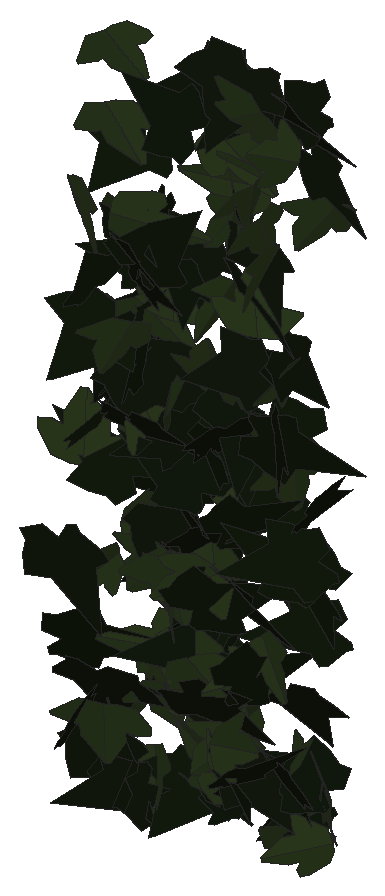
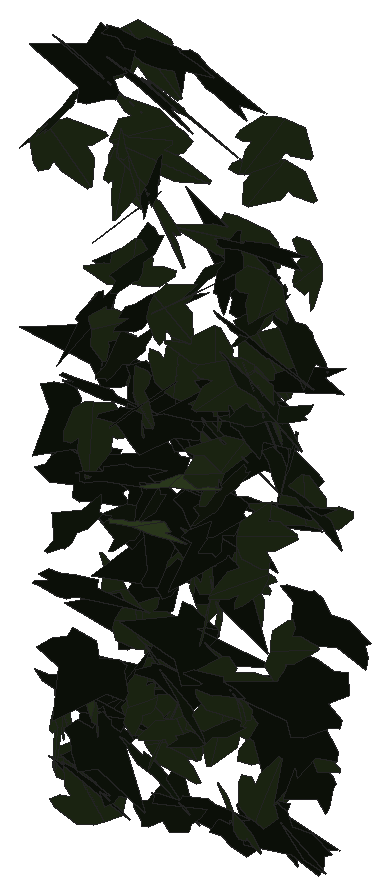
# SketchUp Ruby script. Lengths in inches.
U = 1.inch
M = Sketchup.active_model
def pt(a) = Geom::Point3d.new(a.map { |v| v * U })
def face(e, loops, mat)
  f = e.add_face(loops[0].map { |a| pt(a) })
  loops[1..].each { |l| e.add_face(l.map { |a| pt(a) }).erase! }
  f.material = f.back_material = mat if mat
  f
end
# faces: each face lists its corners as indices into pts; further lists are holes
def faces(e, pts, list, mat = nil) = list.each { |f| face(e, (f[0].is_a?(Array) ? f : [f]).map { |l| l.map { |i| pts[i] } }, mat) }
# xy, xz, yz: faces in a plane at the given z, y or x. An outline is a flat list of corners, or four numbers for a rectangle; further outlines are holes
def ring(l) = l.size == 4 ? [[l[0], l[1]], [l[2], l[1]], [l[2], l[3]], [l[0], l[3]]] : l.each_slice(2).to_a
def flat(e, list, mat, &to3) = list.each { |f| face(e, (f[0].is_a?(Array) ? f : [f]).map { |l| ring(l).map { |u, v| to3.(u, v) } }, mat) }
def xy(e, z, list, mat = nil) = flat(e, list, mat) { |x, y| [x, y, z] }
def xz(e, y, list, mat = nil) = flat(e, list, mat) { |x, z| [x, y, z] }
def yz(e, x, list, mat = nil) = flat(e, list, mat) { |y, z| [x, y, z] }
def lines(e, pts, list) = list.each { |a, b| e.add_line(pt(pts[a]), pt(pts[b])) }
# prism: a flat outline (further loops are holes) pulled along v
def prism(e, loops, v, mat = nil)
  f = face(e, loops, mat); d = Geom::Vector3d.new(v.map { |x| x * U })
  f.pushpull(f.normal.samedirection?(d) ? d.length : -d.length)
end
def box(e, o, s, mat = nil) = prism(e, [[o, [o[0] + s[0], o[1], o[2]], [o[0] + s[0], o[1] + s[1], o[2]], [o[0], o[1] + s[1], o[2]]]], [0, 0, s[2]], mat)
def at(x, y, z, deg = 0) = Geom::Transformation.translation(pt([x, y, z])) * Geom::Transformation.rotation(ORIGIN, Z_AXIS, deg.degrees)
def axes(o, x, y, z) = Geom::Transformation.new([*x, 0, *y, 0, *z, 0, *pt(o).to_a, 1])
def part(name) = M.definitions.add(name)
# library, detail: a bought-in or finely detailed component or shape, given as its bounding box
def library(name, o, s) = part(name).tap { |d| box(d.entities, o, s) }
def detail(e, o, s) = box(e.add_group.entities, o, s)
def put(e, d, t, mat = nil) = e.add_instance(d, t).tap { |i| i.material = mat if mat }
def group(e, t, mat = nil) = e.add_group.tap { |g| g.transformation = t; g.material = mat if mat }.entities
root = M.entities
M.materials.add("1026 AP 7946 SUNNY SIDE UP").color = [254, 231, 186]
M.materials.add("efeu1").color = [18, 25, 13]
M.materials.add("efeu2").color = [43, 57, 29]
c1 = part("ivyleaf_9")
p = [[1.54,2.16,1.25],[1.36,2.04,1.19],[-0.21,0.99,0.68],[-0.71,1.11,0.82],[-0.85,0.86,0.67],[-0.8,0.17,0.21],
  [-0.9,-0.01,0.1],[-0.67,-0.16,-0.02],[-0.08,-0.08,-0.05],[-0.03,-0.6,-0.4],[0.65,-0.88,-0.66],[0.83,-0.6,-0.49],
  [1.29,-0.42,-0.43],[1.8125,-0.07,-0.26],[1.21,0.44,0.15]]
faces(c1.entities,p,[[0,1,2,3,4,5,6,7,8,9,10,11,12,13,14]],"efeu1")
c2 = part("ivyleaf_10")
p = [[0,0.5,-0.03],[-0.0625,2.02,-0.43],[-0.19,2.01,-0.46],[-0.54,1.05,-0.29],[-0.52,0.625,-0.18],[-0.83,0.76,-0.28],
  [-1.16,0.64,-0.33],[-1.15,0.33,-0.24],[-0.77,-0.39,0.02],[-0.3,-0.51,0.16],[0.04,-0.48,0.23],[-0.02,2.01,-0.4375],
  [-0.06,2.01,-0.43],[0.04,-0.49,0.23],[0.67,-0.49,0.14],[1.38,0.36,-0.2],[1.375,0.51,-0.24],[0.81,0.65,-0.19],
  [0.62,0.59,-0.15],[0.6,1.09,-0.28],[0.5,1.23,-0.31]]
faces(c2.entities,p,[[0,1,2,3,4,5,6,7,8,9,10],[11,12,0,13,14,15,16,17,18,19,20]],"efeu2")
put(root,c1,axes([144.02,211.13,286.05],[0.051,-0.0466,-0.38106],[0.48121,-0.20826,0.05349],[-0.33408,-0.30709,0.01888]),"1026 AP 7946 SUNNY SIDE UP")
put(root,c1,axes([142.66,210.79,290.45],[-0.41002,0.00525,-0.29295],[-0.44658,0.01655,0.26868],[0.02475,0.38549,-0.00529]),"1026 AP 7946 SUNNY SIDE UP")
put(root,c2,axes([143.42,210.64,280.99],[-0.03526,0.16378,0.34753],[-0.07787,0.33276,-0.16835],[-0.58316,-0.05434,0.00147]),"1026 AP 7946 SUNNY SIDE UP")
put(root,c2,axes([143.85,211.09,288.69],[0.13652,-0.34131,0.17691],[0.06301,-0.169,-0.3638],[0.59885,0.09559,-0.00205]),"1026 AP 7946 SUNNY SIDE UP")
put(root,c1,axes([143.42,210.74,280.36],[0.16891,0.33769,-0.08584],[0.01032,0.08722,0.36501],[0.54754,-0.10582,0.0196]),"1026 AP 7946 SUNNY SIDE UP")
put(root,c2,axes([141.375,211.02,286.71],[-0.25952,-0.30703,0.11261],[-0.06423,-0.10404,-0.35948],[0.50935,-0.16955,0.01205]),"1026 AP 7946 SUNNY SIDE UP")
put(root,c2,axes([144.08,211.18,290.28],[-0.01561,0.17803,0.34127],[0.06022,-0.32817,0.18151],[0.58687,0.03841,-0.00955]),"1026 AP 7946 SUNNY SIDE UP")
put(root,c2,axes([141.08,210.96,280.56],[-0.55199,-0.18292,0.00641],[0.01698,-0.03637,-0.4062],[0.28735,-0.34923,0.03632]),"1026 AP 7946 SUNNY SIDE UP")
put(root,c1,axes([143.14,211.19,280.37],[0.06729,-0.26436,0.21998],[0.07612,-0.20981,-0.27687],[0.53039,0.06365,0.01183]),"1026 AP 7946 SUNNY SIDE UP")
put(root,c1,axes([140.21,211.05,282.93],[-0.25952,-0.09043,-0.37086],[0.54319,0.10514,-0.19003],[0.21132,-0.38132,0.03302]),"1026 AP 7946 SUNNY SIDE UP")
put(root,c1,axes([141.36,211.19,287.61],[0.18886,-0.16012,0.31476],[0.21959,-0.2743,-0.20565],[0.49735,0.18192,-0.02872]),"1026 AP 7946 SUNNY SIDE UP")
put(root,c2,axes([142.77,211.04,283.27],[0.43211,-0.0276,-0.24252],[-0.37047,0.00526,-0.28414],[0.03836,0.36171,-0.01225]),"1026 AP 7946 SUNNY SIDE UP")
put(root,c1,axes([142.77,210.87,282.84],[0.00919,0.02174,0.39223],[0.59548,0.04342,-0.00829],[-0.06889,0.37817,-0.01935]),"1026 AP 7946 SUNNY SIDE UP")
put(root,c2,axes([141.98,211.29,282.53],[0.00162,-0.02873,-0.38292],[0.14518,-0.35993,0.02683],[-0.56767,-0.09213,0.00577]),"1026 AP 7946 SUNNY SIDE UP")
put(root,c1,axes([142.73,210.95,284.68],[-0.10724,0.15198,0.33389],[-0.479,0.14708,-0.1366],[-0.29327,-0.29581,0.10101]),"1026 AP 7946 SUNNY SIDE UP")
put(root,c1,axes([140.63,210.72,280.29],[0.06819,0.18704,0.34131],[0.17457,0.3116,-0.19501],[-0.57067,0.11767,-0.01887]),"1026 AP 7946 SUNNY SIDE UP")
put(root,c1,axes([140.89,211.33,286.51],[-0.40385,-0.2696,0.15117],[-0.13022,-0.12544,-0.38349],[0.46594,-0.26873,0.02385]),"1026 AP 7946 SUNNY SIDE UP")
put(root,c1,axes([144.55,211.23,284.06],[-0.48677,-0.03035,0.18876],[-0.27841,-0.06036,-0.31854],[0.08903,-0.35472,0.03591]),"1026 AP 7946 SUNNY SIDE UP")
put(root,c2,axes([143.46,211.32,281.8125],[-0.12307,-0.01797,0.34416],[-0.11811,-0.3335,-0.03855],[0.5128,-0.08112,0.07372]),"1026 AP 7946 SUNNY SIDE UP")
put(root,c1,axes([141.66,211.03,287.88],[-0.264,0.21162,0.30055],[0.33459,-0.19993,0.27552],[0.4555,0.2695,-0.02819]),"1026 AP 7946 SUNNY SIDE UP")
put(root,c1,axes([143.41,211.36,286.61],[-0.23239,-0.10983,0.32218],[-0.32126,-0.2403,-0.18744],[0.41158,-0.24958,0.0356]),"1026 AP 7946 SUNNY SIDE UP")
put(root,c1,axes([142.57,210.93,281.4],[0.55612,0.11164,0.10887],[0.17566,-0.00682,-0.38004],[-0.16506,0.36889,-0.03762]),"1026 AP 7946 SUNNY SIDE UP")
put(root,c1,axes([141.49,211.3,279.44],[-0.04792,-0.05968,-0.36006],[-0.17902,-0.33021,0.06645],[-0.52743,0.1175,0.01016]),"1026 AP 7946 SUNNY SIDE UP")
put(root,c2,axes([142.125,211.13,283.13],[-0.58142,-0.15639,-0.04207],[0.10036,-0.04996,-0.40746],[0.23312,-0.36855,0.0705]),"1026 AP 7946 SUNNY SIDE UP")
put(root,c1,axes([143.48,211.08,280.49],[0.07023,-0.24147,-0.25612],[-0.02756,0.24739,-0.25073],[0.54272,0.04381,0.02041]),"1026 AP 7946 SUNNY SIDE UP")
put(root,c1,axes([142.32,211.14,285.36],[-0.46374,0.23477,0.0162],[-0.04516,-0.01304,-0.38734],[-0.36708,-0.29499,0.02719]),"1026 AP 7946 SUNNY SIDE UP")
put(root,c1,axes([140.38,210.98,281.5],[0.28045,0.07021,0.36112],[0.54911,0.04756,-0.1928],[-0.11743,0.39006,-0.03911]),"1026 AP 7946 SUNNY SIDE UP")
put(root,c1,axes([143.77,211.09,285.82],[0.25466,-0.00531,-0.33978],[0.39086,0.24346,0.12314],[0.3409,-0.27518,0.11263]),"1026 AP 7946 SUNNY SIDE UP")
put(root,c2,axes([140.34,211.27,288.4375],[-0.29347,0.24032,-0.2328],[0.17324,-0.20097,-0.31322],[-0.49048,-0.21478,0.02867]),"1026 AP 7946 SUNNY SIDE UP")
put(root,c1,axes([143.08,211.11,285.68],[-0.02537,0.337,-0.14455],[0.02424,-0.14162,-0.3483],[-0.57465,-0.02085,-0.00831]),"1026 AP 7946 SUNNY SIDE UP")
put(root,c1,axes([141.52,211.01,285.35],[0.61771,0.06958,-0.10511],[-0.16737,0.0157,-0.40951],[-0.09946,0.40567,0.03632]),"1026 AP 7946 SUNNY SIDE UP")
put(root,c1,axes([140.87,211.11,285.11],[-0.26971,0.33859,-0.04449],[0.00492,-0.04892,-0.3908],[-0.53708,-0.17048,0.01877]),"1026 AP 7946 SUNNY SIDE UP")
put(root,c1,axes([140.87,211.07,281.08],[0.50651,0.17273,-0.1679],[-0.21959,-0.08641,-0.37693],[-0.30334,0.35097,-0.0075]),"1026 AP 7946 SUNNY SIDE UP")
put(root,c2,axes([141.87,211.23,283.17],[-0.50382,-0.04345,0.19818],[-0.28559,-0.07919,-0.33012],[0.12181,-0.36537,0.04571]),"1026 AP 7946 SUNNY SIDE UP")
put(root,c2,axes([143.58,211.33,282.29],[0.32351,-0.07386,0.27122],[0.38296,-0.10143,-0.22562],[0.19684,0.31871,-0.0068]),"1026 AP 7946 SUNNY SIDE UP")
put(root,c2,axes([142.6875,211.27,283.47],[0.53836,-0.02327,0.11009],[0.16537,-0.02786,-0.35311],[0.04791,0.35762,-0.01824]),"1026 AP 7946 SUNNY SIDE UP")
put(root,c2,axes([143.51,211.18,290.8],[-0.37943,0.02082,0.30069],[-0.45991,-0.02122,-0.24777],[0.00492,-0.37802,0.02824]),"1026 AP 7946 SUNNY SIDE UP")
put(root,c2,axes([143.08,211.34,280.67],[-0.35285,-0.16502,0.22702],[-0.20863,-0.18562,-0.28228],[0.38065,-0.25471,0.05572]),"1026 AP 7946 SUNNY SIDE UP")
put(root,c2,axes([144.41,211.46,279.41],[-0.10226,0.00253,0.34629],[-0.12064,-0.33343,-0.01466],[0.51459,-0.07767,0.06538]),"1026 AP 7946 SUNNY SIDE UP")
put(root,c2,axes([142.55,211.19,281.69],[-0.45704,-0.11165,-0.21684],[0.33498,0.02467,-0.31737],[0.16578,-0.35765,0.04349]),"1026 AP 7946 SUNNY SIDE UP")
put(root,c1,axes([141.97,211.5,287.78],[-0.00831,-0.32593,0.16601],[0.01055,-0.16307,-0.33666],[0.5729,-0.00172,0.0086]),"1026 AP 7946 SUNNY SIDE UP")
put(root,c1,axes([144.41,211.3125,283.64],[-0.0171,0.06942,0.37548],[-0.58225,0.01365,-0.01399],[-0.02509,-0.36398,0.06888]),"1026 AP 7946 SUNNY SIDE UP")
put(root,c2,axes([142.18,211.01,285.72],[0.15723,-0.04257,0.3662],[-0.32599,0.2943,0.09805],[-0.4594,-0.22341,0.05575]),"1026 AP 7946 SUNNY SIDE UP")
put(root,c1,axes([142.76,211.16,285.22],[0.05396,-0.00324,-0.36796],[-0.56156,-0.00564,-0.03533],[-0.00834,0.35876,-0.00178]),"1026 AP 7946 SUNNY SIDE UP")
put(root,c1,axes([143.35,211,281.8],[0.05904,0.07713,0.3889],[0.50163,0.2057,-0.07487],[-0.33855,0.31824,-0.04312]),"1026 AP 7946 SUNNY SIDE UP")
put(root,c1,axes([142.52,211.46,281.875],[-0.0717,-0.11857,-0.3305],[-0.20961,-0.29116,0.12895],[-0.49419,0.1407,-0.00674]),"1026 AP 7946 SUNNY SIDE UP")
put(root,c1,axes([141.24,211.27,284.28],[-0.4652,-0.17399,-0.0994],[-0.15413,-0.02097,0.35207],[-0.27137,0.31018,-0.02956]),"1026 AP 7946 SUNNY SIDE UP")
put(root,c1,axes([142.75,211.1875,283.95],[0.06618,0.33439,-0.1291],[-0.01721,-0.12683,-0.34791],[-0.56229,0.04324,-0.00455]),"1026 AP 7946 SUNNY SIDE UP")
put(root,c2,axes([142.97,211.24,279.98],[-0.07722,0.39391,-0.00226],[0.00645,0.00498,0.40894],[0.61939,0.04905,-0.00454]),"1026 AP 7946 SUNNY SIDE UP")
put(root,c2,axes([141.33,211.23,288.39],[-0.04543,-0.0261,-0.40547],[0.61934,0.01633,-0.03082],[0.02867,-0.39416,0.02325]),"1026 AP 7946 SUNNY SIDE UP")
put(root,c1,axes([143.89,211.24,280.55],[0.4845,-0.10162,-0.14324],[-0.22619,0.00272,-0.3318],[0.14758,0.3378,-0.03827]),"1026 AP 7946 SUNNY SIDE UP")
put(root,c2,axes([140.5,211.2,284.4375],[0.53923,0.21013,-0.0385],[0.0204,0.05231,0.41282],[0.33531,-0.34111,0.0368]),"1026 AP 7946 SUNNY SIDE UP")
put(root,c1,axes([143.08,211.1,284.08],[0.0469,0.02991,0.35185],[0.47544,0.15895,-0.04063],[-0.25357,0.30357,-0.01111]),"1026 AP 7946 SUNNY SIDE UP")
put(root,c1,axes([140.85,211.01,287.25],[-0.00642,0.31856,0.26985],[-0.06591,0.25846,-0.32525],[-0.64333,-0.02966,0.03063]),"1026 AP 7946 SUNNY SIDE UP")
put(root,c2,axes([143.01,211.23,280.07],[-0.34385,0.07316,-0.33261],[-0.44514,0.16021,0.23556],[0.27107,0.35589,-0.03508]),"1026 AP 7946 SUNNY SIDE UP")
put(root,c2,axes([142.11,211.38,281.88],[0.44987,0.02204,0.22094],[0.33877,-0.03491,-0.29276],[0.00537,0.35578,-0.04031]),"1026 AP 7946 SUNNY SIDE UP")
put(root,c1,axes([141.99,211.27,283.11],[0.16238,0.05066,-0.35441],[-0.51662,-0.10422,-0.11793],[-0.18043,0.34402,0.0187]),"1026 AP 7946 SUNNY SIDE UP")
put(root,c1,axes([141.19,211.2,279.49],[-0.27982,0.01122,-0.32514],[-0.49487,0.02466,0.18382],[0.04244,0.36154,-0.00032]),"1026 AP 7946 SUNNY SIDE UP")
put(root,c1,axes([142.75,211.32,283.08],[0.52171,-0.11935,0.08438],[0.10698,-0.05414,-0.36249],[0.20159,0.3376,-0.02602]),"1026 AP 7946 SUNNY SIDE UP")
put(root,c2,axes([143.35,211.3,289.46],[-0.10227,-0.36453,-0.09857],[0.01663,0.09319,-0.38087],[0.59155,-0.06564,-0.00633]),"1026 AP 7946 SUNNY SIDE UP")
put(root,c2,axes([141.47,211.5625,281.43],[-0.16097,-0.03073,-0.33666],[0.2448,-0.30572,-0.02243],[-0.45406,-0.15393,0.10726]),"1026 AP 7946 SUNNY SIDE UP")
put(root,c1,axes([141.39,211.1,285.83],[0.05535,0.05877,0.38859],[-0.03951,0.378,-0.05609],[-0.59844,-0.01952,0.03964]),"1026 AP 7946 SUNNY SIDE UP")
put(root,c2,axes([140.875,211.39,289.8],[-0.46187,-0.14137,-0.13593],[0.25038,-0.04303,-0.31987],[0.17102,-0.31879,0.10119]),"1026 AP 7946 SUNNY SIDE UP")
put(root,c1,axes([141.66,211.62,283.98],[0.13639,-0.18769,0.30475],[0.18906,-0.27147,-0.21458],[0.51893,0.14823,-0.00193]),"1026 AP 7946 SUNNY SIDE UP")
put(root,c1,axes([143.05,211.59,291.125],[-0.57566,-0.14397,-0.13555],[0.21247,0.01216,-0.40348],[0.21995,-0.38856,0.035]),"1026 AP 7946 SUNNY SIDE UP")
put(root,c2,axes([140.65,211.64,282.52],[0.01769,0.11224,-0.32719],[-0.19676,-0.29433,-0.11322],[-0.49279,0.12155,0.03346]),"1026 AP 7946 SUNNY SIDE UP")
put(root,c1,axes([142.875,211.7,285.63],[-0.06354,-0.3982,0.12132],[-0.0195,-0.11938,-0.41302],[0.65366,-0.04227,-0.00053]),"1026 AP 7946 SUNNY SIDE UP")
put(root,c2,axes([143.5,211.34,288.99],[-0.11298,-0.33498,-0.17481],[0.08331,0.16004,-0.35161],[0.58319,-0.08776,0.01636]),"1026 AP 7946 SUNNY SIDE UP")
put(root,c2,axes([141.74,211.63,281.52],[0.04735,0.07295,0.39459],[-0.34418,-0.31425,0.07763],[0.50659,-0.22032,0.01586]),"1026 AP 7946 SUNNY SIDE UP")
put(root,c1,axes([140.54,211.5,279.72],[-0.15834,-0.11435,-0.36878],[0.52328,0.14358,-0.14311],[0.27235,-0.34235,0.06058]),"1026 AP 7946 SUNNY SIDE UP")
put(root,c1,axes([143.2,211.32,279.78],[-0.22871,0.27485,0.14026],[-0.16319,0.09589,-0.31672],[-0.4527,-0.17343,0.04331]),"1026 AP 7946 SUNNY SIDE UP")
put(root,c2,axes([141.6,211.35,285.19],[0.24986,0.33106,0.13706],[0.09988,0.11497,-0.37756],[-0.55094,0.17099,-0.00629]),"1026 AP 7946 SUNNY SIDE UP")
put(root,c1,axes([142.79,211.31,282.89],[-0.09054,-0.15315,0.32786],[0.33347,0.24394,0.16145],[-0.44563,0.21366,0.0542]),"1026 AP 7946 SUNNY SIDE UP")
put(root,c2,axes([143.08,211.73,280.88],[0.00484,0.07556,-0.37536],[-0.14634,-0.35308,-0.07822],[-0.5672,0.09174,0.01698]),"1026 AP 7946 SUNNY SIDE UP")
put(root,c1,axes([141.33,211.33,286.04],[0.16389,-0.16952,-0.39179],[0.24798,0.37797,-0.12715],[0.60444,-0.1091,0.1584]),"1026 AP 7946 SUNNY SIDE UP")
put(root,c2,axes([143.73,211.72,286.52],[-0.11059,0.09845,-0.34105],[-0.14968,-0.33085,-0.08232],[-0.52293,0.07388,0.09569]),"1026 AP 7946 SUNNY SIDE UP")
put(root,c2,axes([141.75,211.45,281],[-0.34505,-0.2505,-0.08079],[0.10243,0.04514,-0.34227],[0.39914,-0.22814,0.01799]),"1026 AP 7946 SUNNY SIDE UP")
put(root,c1,axes([144.5,211.43,280.375],[-0.27519,0.15239,0.29296],[-0.41616,0.11552,-0.2316],[-0.28802,-0.31251,0.05473]),"1026 AP 7946 SUNNY SIDE UP")
put(root,c1,axes([141.74,211.34,283.86],[0.04925,-0.19291,-0.34576],[-0.08218,0.33043,-0.1994],[0.60163,0.06093,0.00106]),"1026 AP 7946 SUNNY SIDE UP")
put(root,c2,axes([141.35,211.64,279.65],[0.3925,-0.13871,0.22623],[0.26912,-0.14269,-0.29306],[0.30859,0.30086,-0.03217]),"1026 AP 7946 SUNNY SIDE UP")
put(root,c1,axes([142.78,211.77,288.89],[-0.01028,-0.04722,0.38112],[-0.02286,-0.36996,-0.05105],[0.58641,-0.01525,0.00469]),"1026 AP 7946 SUNNY SIDE UP")
put(root,c1,axes([142.23,211.7,279.61],[-0.51481,-0.1495,-0.01446],[0.03993,-0.02399,-0.36943],[0.23259,-0.32679,0.03141]),"1026 AP 7946 SUNNY SIDE UP")
put(root,c1,axes([141.25,211.7,286.125],[-0.35429,0.10957,-0.26929],[0.24121,-0.23452,-0.2383],[-0.37582,-0.25381,0.10091]),"1026 AP 7946 SUNNY SIDE UP")
put(root,c1,axes([143.18,211.7,288.43],[0.08584,-0.36796,0.01992],[-0.0033,-0.02197,-0.38331],[0.57955,0.05437,-0.00513]),"1026 AP 7946 SUNNY SIDE UP")
put(root,c1,axes([143,211.6875,287.76],[0.26216,-0.30471,0.11327],[0.07591,-0.10087,-0.35837],[0.50462,0.17348,-0.00494]),"1026 AP 7946 SUNNY SIDE UP")
put(root,c2,axes([143.33,211.46,287.32],[0.44377,0.22803,-0.01343],[-0.01209,0.03224,0.37271],[0.35906,-0.28074,0.02915]),"1026 AP 7946 SUNNY SIDE UP")
put(root,c2,axes([143.15,211.55,289.39],[0.11412,-0.01954,-0.37672],[-0.57044,0.04612,-0.07647],[0.07716,0.36984,-0.00816]),"1026 AP 7946 SUNNY SIDE UP")
put(root,c2,axes([142.46,211.57,286],[-0.55879,0.07283,0.00569],[0.01663,0.02623,0.37276],[0.11359,0.35444,-0.02658]),"1026 AP 7946 SUNNY SIDE UP")
put(root,c1,axes([142.51,211.79,279.3],[-0.29881,-0.11665,0.21323],[0.15892,-0.28003,-0.06841],[0.33909,0.02846,0.21996]),"1026 AP 7946 SUNNY SIDE UP")
put(root,c2,axes([140.96,211.61,286.47],[0.2475,-0.32145,-0.03347],[-0.05134,0.0181,-0.36796],[0.50514,0.15934,-0.021]),"1026 AP 7946 SUNNY SIDE UP")
put(root,c1,axes([140.32,211.86,285.48],[0.14373,-0.16966,-0.31945],[0.40744,-0.18428,0.18205],[-0.37607,-0.2645,0.07515]),"1026 AP 7946 SUNNY SIDE UP")
put(root,c2,axes([142.72,211.55,289.91],[0.36052,0.10019,0.28471],[0.41221,0.08731,-0.25668],[-0.20729,0.34787,-0.01524]),"1026 AP 7946 SUNNY SIDE UP")
put(root,c1,axes([142.94,211.77,283.79],[0.23117,-0.32702,0.12823],[0.0777,-0.11629,-0.37004],[0.54573,0.15508,-0.00163]),"1026 AP 7946 SUNNY SIDE UP")
put(root,c1,axes([141.4,211.83,288.35],[-0.08349,0.02961,-0.38672],[0.41402,-0.26833,-0.06171],[-0.42364,-0.26807,0.0159]),"1026 AP 7946 SUNNY SIDE UP")
put(root,c1,axes([141.92,211.59,284.37],[0.03254,0.03646,-0.36137],[-0.49739,-0.1539,-0.03658],[-0.2459,0.31612,0.02618]),"1026 AP 7946 SUNNY SIDE UP")
put(root,c1,axes([144.02,211.8125,283.26],[0.07951,-0.29338,0.17226],[0.0944,-0.16027,-0.3063],[0.52385,0.07341,0.02905]),"1026 AP 7946 SUNNY SIDE UP")
put(root,c2,axes([141.98,211.4375,282.45],[-0.05873,0.31928,-0.18854],[-0.02374,0.1843,0.33219],[0.57961,0.0399,-0.0055]),"1026 AP 7946 SUNNY SIDE UP")
put(root,c1,axes([142.8125,211.74,285.41],[-0.31,-0.25942,-0.17623],[0.20745,0.11163,-0.33327],[0.44099,-0.23488,0.03289]),"1026 AP 7946 SUNNY SIDE UP")
put(root,c2,axes([140.83,211.85,280.08],[-0.09547,-0.23564,-0.27663],[-0.11206,-0.25753,0.24916],[-0.54885,0.09357,-0.00275]),"1026 AP 7946 SUNNY SIDE UP")
put(root,c2,axes([144.59,211.45,280.13],[-0.24183,0.26655,0.23286],[-0.23833,0.16983,-0.31368],[-0.49346,-0.21265,0.03738]),"1026 AP 7946 SUNNY SIDE UP")
put(root,c1,axes([144.39,211.33,284.72],[0.11147,0.23196,0.28815],[0.18773,0.25287,-0.2469],[-0.53796,0.13631,-0.02645]),"1026 AP 7946 SUNNY SIDE UP")
put(root,c1,axes([141.69,211.81,280.875],[0.05488,-0.31337,0.07481],[0.22733,-0.05163,-0.2942],[0.45255,0.06394,0.13871]),"1026 AP 7946 SUNNY SIDE UP")
put(root,c2,axes([142.46,211.85,287.33],[-0.05614,-0.30345,0.21902],[0.04387,-0.2169,-0.31284],[0.58251,-0.01291,0.04467]),"1026 AP 7946 SUNNY SIDE UP")
put(root,c1,axes([143.1,211.77,290.67],[-0.55155,0.05026,-0.09198],[0.12999,-0.05099,-0.36329],[-0.09583,-0.35841,0.0366]),"1026 AP 7946 SUNNY SIDE UP")
put(root,c2,axes([142.28,211.73,280.81],[0.36454,0.23218,-0.11321],[-0.10396,-0.09094,-0.33811],[-0.39121,0.24051,-0.01564]),"1026 AP 7946 SUNNY SIDE UP")
put(root,c1,axes([140.73,211.84,287.74],[0.15453,-0.33589,0.09597],[0.0357,-0.0924,-0.36105],[0.54774,0.10079,-0.00354]),"1026 AP 7946 SUNNY SIDE UP")
put(root,c2,axes([140.88,211.65,288.09],[-0.4996,0.16549,-0.01485],[-0.00108,-0.03444,-0.36789],[-0.26133,-0.31623,0.02991]),"1026 AP 7946 SUNNY SIDE UP")
put(root,c2,axes([142.72,211.67,288.7],[0.3398,-0.27306,-0.13555],[-0.15326,0.0884,-0.35762],[0.45017,0.2362,-0.01944]),"1026 AP 7946 SUNNY SIDE UP")
put(root,c1,axes([143.45,211.79,290.57],[0.32066,-0.17626,0.25433],[0.29999,-0.15829,-0.27858],[0.37246,0.27923,0.00543]),"1026 AP 7946 SUNNY SIDE UP")
put(root,c1,axes([143.41,211.92,284.44],[-0.39748,-0.20662,0.0875],[-0.0629,-0.08609,-0.33431],[0.34631,-0.25279,0.03971]),"1026 AP 7946 SUNNY SIDE UP")
put(root,c2,axes([144.5625,211.45,280.32],[0.06945,-0.00994,-0.38505],[-0.20752,0.35166,-0.02365],[0.54998,0.13394,0.0397]),"1026 AP 7946 SUNNY SIDE UP")
put(root,c2,axes([144.34,211.83,289.28],[-0.27462,-0.27186,0.16814],[-0.12118,-0.14617,-0.33348],[0.48494,-0.19048,0.01189]),"1026 AP 7946 SUNNY SIDE UP")
put(root,c2,axes([143.97,211.51,280.48],[0.20377,-0.02939,0.31263],[-0.29898,0.25019,0.11002],[-0.3751,-0.21539,0.08215]),"1026 AP 7946 SUNNY SIDE UP")
put(root,c2,axes([140.82,212,284.36],[0.01134,-0.07718,0.35533],[-0.0003,-0.34542,-0.08154],[0.55642,0.00139,-0.00729]),"1026 AP 7946 SUNNY SIDE UP")
put(root,c1,axes([143.95,211.8125,285.57],[-0.45268,0.10593,0.17362],[-0.29462,-0.04706,-0.3006],[-0.10332,-0.32995,0.09644]),"1026 AP 7946 SUNNY SIDE UP")
put(root,c1,axes([142.03,211.49,282.02],[0.05199,0.32265,-0.17638],[0.0141,0.17298,0.33505],[0.57552,-0.03338,0.00772]),"1026 AP 7946 SUNNY SIDE UP")
put(root,c1,axes([141.375,211.91,284.77],[0.1783,-0.33908,0.07895],[0.02822,-0.07682,-0.36871],[0.54657,0.11458,-0.00672]),"1026 AP 7946 SUNNY SIDE UP")
put(root,c2,axes([141.84,211.52,284.79],[0.14517,-0.14835,0.33411],[-0.13238,0.31735,0.17564],[-0.54616,-0.11635,0.04623]),"1026 AP 7946 SUNNY SIDE UP")
put(root,c2,axes([143.78,211.73,285.07],[-0.21673,-0.36412,-0.08148],[0.0806,0.06279,-0.39988],[0.57964,-0.14487,0.02513]),"1026 AP 7946 SUNNY SIDE UP")
put(root,c1,axes([143.73,211.64,286.87],[0.18549,-0.18005,-0.29489],[-0.23524,0.24288,-0.22028],[0.47535,0.19046,0.00606]),"1026 AP 7946 SUNNY SIDE UP")
put(root,c2,axes([141.17,211.51,283.4],[0.01834,0.00219,0.36551],[-0.02686,0.35457,0.00039],[-0.55723,-0.01702,0.01201]),"1026 AP 7946 SUNNY SIDE UP")
put(root,c2,axes([143.2,211.54,285.6],[0.02728,-0.00463,-0.40759],[-0.2788,0.35391,-0.0102],[0.55614,0.17765,0.01488]),"1026 AP 7946 SUNNY SIDE UP")
put(root,c1,axes([142.08,211.93,281.75],[-0.3814,-0.23383,-0.14777],[0.19484,0.07545,-0.34534],[0.3836,-0.27081,0.02849]),"1026 AP 7946 SUNNY SIDE UP")
put(root,c1,axes([143.7,211.79,280.22],[-0.16917,0.30676,-0.17196],[0.0487,-0.16741,-0.33501],[-0.54828,-0.10951,0.0233]),"1026 AP 7946 SUNNY SIDE UP")
put(root,c1,axes([141.15,211.67,286.67],[-0.25666,0.31623,0.08709],[-0.11045,0.05639,-0.36445],[-0.50197,-0.1741,0.03566]),"1026 AP 7946 SUNNY SIDE UP")
put(root,c1,axes([140.54,212.02,286.32],[-0.12183,-0.32291,0.06835],[0.28617,-0.10023,-0.27654],[0.4329,-0.02462,0.20205]),"1026 AP 7946 SUNNY SIDE UP")
put(root,c1,axes([144.11,211.84,290.76],[-0.50252,0.15077,0.01278],[-0.03536,-0.02067,-0.36299],[-0.23512,-0.31913,0.02726]),"1026 AP 7946 SUNNY SIDE UP")
put(root,c1,axes([143.62,211.56,279.63],[-0.09629,0.29189,-0.15352],[-0.13624,0.13349,0.30346],[0.49822,0.09292,0.05331]),"1026 AP 7946 SUNNY SIDE UP")
put(root,c2,axes([142.13,212.07,284.73],[-0.46653,-0.11339,0.0872],[0.17511,-0.3086,-0.02538],[0.13824,0.00824,0.32642]),"1026 AP 7946 SUNNY SIDE UP")
put(root,c1,axes([142.02,211.8,281.08],[-0.08079,0.29727,0.19031],[0.06444,-0.1786,0.30962],[0.54514,0.06517,-0.0084]),"1026 AP 7946 SUNNY SIDE UP")
put(root,c2,axes([143.67,211.83,279.07],[-0.27392,-0.2929,0.10273],[0.07532,0.08947,0.35157],[-0.48151,0.18062,-0.00345]),"1026 AP 7946 SUNNY SIDE UP")
put(root,c2,axes([140.54,211.78,290.7],[-0.29831,-0.25537,-0.17725],[0.25781,0.08534,-0.31894],[0.40833,-0.24045,0.07188]),"1026 AP 7946 SUNNY SIDE UP")
put(root,c1,axes([144.05,211.87,289.96],[0.29977,-0.28777,-0.14545],[-0.1079,0.12188,-0.35477],[0.49118,0.2024,0.01084]),"1026 AP 7946 SUNNY SIDE UP")
put(root,c2,axes([141.12,211.83,286.64],[-0.41372,-0.12278,-0.22154],[0.33908,0.03859,-0.29524],[0.18947,-0.33717,0.04463]),"1026 AP 7946 SUNNY SIDE UP")
put(root,c1,axes([141.82,212.12,287.83],[-0.09432,-0.33784,0.09234],[0.03876,-0.09673,-0.35166],[0.54901,-0.05121,0.04069]),"1026 AP 7946 SUNNY SIDE UP")
put(root,c1,axes([144.2,212.04,282.5],[-0.4424,-0.01208,0.18616],[-0.27834,-0.05282,-0.28777],[0.06069,-0.33022,0.03724]),"1026 AP 7946 SUNNY SIDE UP")
put(root,c1,axes([142.93,212.17,286.43],[-0.0385,-0.25325,0.23809],[0.0543,-0.23377,-0.25988],[0.53789,0.00547,0.04328]),"1026 AP 7946 SUNNY SIDE UP")
put(root,c1,axes([142.49,211.9,290.69],[-0.45137,0.2137,0.06882],[-0.13152,-0.00368,-0.36478],[-0.32596,-0.29443,0.05188]),"1026 AP 7946 SUNNY SIDE UP")
put(root,c1,axes([141.19,211.85,287.38],[-0.33594,0.20329,0.17722],[-0.24606,0.08082,-0.30014],[-0.33738,-0.26137,0.04243]),"1026 AP 7946 SUNNY SIDE UP")
put(root,c2,axes([142.65,212.17,283.95],[-0.50953,-0.01628,0.01491],[0.02342,-0.32307,-0.03252],[0.02512,-0.029,0.33267]),"1026 AP 7946 SUNNY SIDE UP")
put(root,c2,axes([141.57,211.86,286.79],[0.53439,0.09764,0.01601],[-0.04233,0.03988,0.36146],[0.14946,-0.33784,0.04513]),"1026 AP 7946 SUNNY SIDE UP")
put(root,c1,axes([143.96,212.03,279.66],[-0.47091,0.05069,-0.0269],[0.03291,-0.03375,-0.31161],[-0.08362,-0.29874,0.02882]),"1026 AP 7946 SUNNY SIDE UP")
put(root,c1,axes([143.63,211.85,281.4],[0.51459,0.08865,-0.06837],[-0.08612,-0.05218,-0.34769],[-0.1519,0.32992,-0.0345]),"1026 AP 7946 SUNNY SIDE UP")
put(root,c1,axes([140.76,212.18,289.03],[-0.47824,-0.1699,0.01607],[0.03606,-0.07421,-0.35072],[0.26599,-0.29542,0.07645]),"1026 AP 7946 SUNNY SIDE UP")
